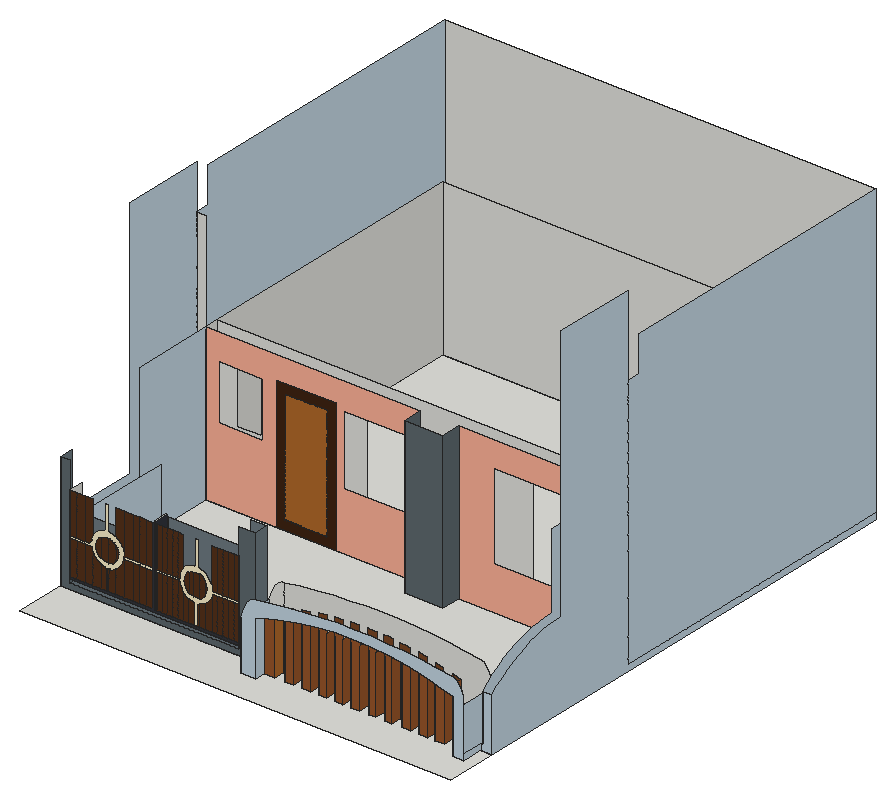
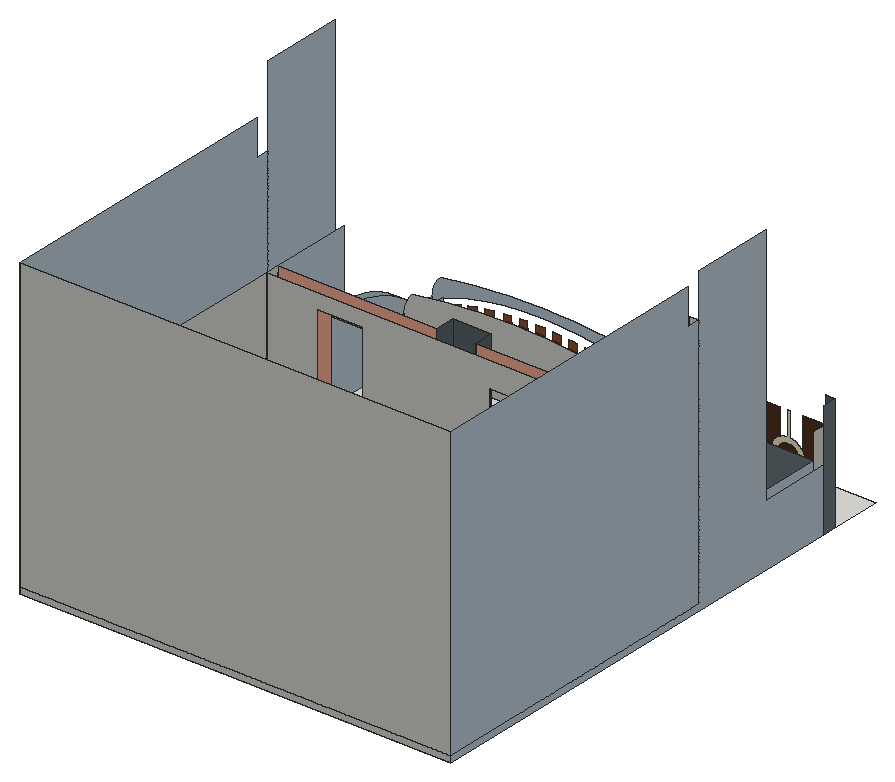
# SketchUp Ruby script. Lengths in inches.
U = 1.inch
M = Sketchup.active_model
def pt(a) = Geom::Point3d.new(a.map { |v| v * U })
def face(e, loops, mat)
  f = e.add_face(loops[0].map { |a| pt(a) })
  loops[1..].each { |l| e.add_face(l.map { |a| pt(a) }).erase! }
  f.material = f.back_material = mat if mat
  f
end
# faces: each face lists its corners as indices into pts; further lists are holes
def faces(e, pts, list, mat = nil) = list.each { |f| face(e, (f[0].is_a?(Array) ? f : [f]).map { |l| l.map { |i| pts[i] } }, mat) }
# xy, xz, yz: faces in a plane at the given z, y or x. An outline is a flat list of corners, or four numbers for a rectangle; further outlines are holes
def ring(l) = l.size == 4 ? [[l[0], l[1]], [l[2], l[1]], [l[2], l[3]], [l[0], l[3]]] : l.each_slice(2).to_a
def flat(e, list, mat, &to3) = list.each { |f| face(e, (f[0].is_a?(Array) ? f : [f]).map { |l| ring(l).map { |u, v| to3.(u, v) } }, mat) }
def xy(e, z, list, mat = nil) = flat(e, list, mat) { |x, y| [x, y, z] }
def xz(e, y, list, mat = nil) = flat(e, list, mat) { |x, z| [x, y, z] }
def yz(e, x, list, mat = nil) = flat(e, list, mat) { |y, z| [x, y, z] }
def lines(e, pts, list) = list.each { |a, b| e.add_line(pt(pts[a]), pt(pts[b])) }
# prism: a flat outline (further loops are holes) pulled along v
def prism(e, loops, v, mat = nil)
  f = face(e, loops, mat); d = Geom::Vector3d.new(v.map { |x| x * U })
  f.pushpull(f.normal.samedirection?(d) ? d.length : -d.length)
end
def box(e, o, s, mat = nil) = prism(e, [[o, [o[0] + s[0], o[1], o[2]], [o[0] + s[0], o[1] + s[1], o[2]], [o[0], o[1] + s[1], o[2]]]], [0, 0, s[2]], mat)
def at(x, y, z, deg = 0) = Geom::Transformation.translation(pt([x, y, z])) * Geom::Transformation.rotation(ORIGIN, Z_AXIS, deg.degrees)
def axes(o, x, y, z) = Geom::Transformation.new([*x, 0, *y, 0, *z, 0, *pt(o).to_a, 1])
def part(name) = M.definitions.add(name)
# library, detail: a bought-in or finely detailed component or shape, given as its bounding box
def library(name, o, s) = part(name).tap { |d| box(d.entities, o, s) }
def detail(e, o, s) = box(e.add_group.entities, o, s)
def put(e, d, t, mat = nil) = e.add_instance(d, t).tap { |i| i.material = mat if mat }
def group(e, t, mat = nil) = e.add_group.tap { |g| g.transformation = t; g.material = mat if mat }.entities
root = M.entities
M.materials.add("[Color B02]").color = [255, 178, 153]
M.materials.add("[Color D01]").color = [255, 242, 204]
M.materials.add("[Formica Laminate Dark]").color = [50, 53, 60]
M.materials.add("[Formica Speckled Grey]").color = [110, 123, 130]
M.materials.add("[Formica Speckled Grey]1").color = [94, 105, 111]
M.materials.add("[Terrazzo Light Blue]").color = [196, 214, 227]
M.materials.add("[Wood Bamboo]").color = [177, 105, 43]
M.materials.add("[Wood Cherry Original]").color = [152, 86, 42]
M.materials.add("[Wood Veneer 01]1").color = [86, 50, 26]
M.materials.add("[Wood Veneer 01]2").color = [63, 37, 19]
M.materials.add("[Wood Veneer 01]3").color = [120, 70, 37]
xy(root,0,[[0,0,0,105.19,405.48,105.19,405.48,61.94,435.4375,61.94,435.4375,84.44,457.01,84.44,457.01,105.19,477.51,105.19,477.51,84.44,495.83,84.44,495.83,105.19,513.14,105.19,513.14,84.44,530.58,84.44,530.58,105.19,547.58,105.19,547.58,84.44,564.14,84.44,564.14,105.19,580.83,105.19,580.83,84.44,597.64,84.44,597.64,105.19,613.45,105.19,613.45,84.44,631.83,84.44,631.83,105.19,650.26,105.19,650.26,84.44,665.7,84.44,665.7,105.19,683.14,105.19,683.14,84.44,698.33,84.44,698.33,105.19,718.2,105.19,718.2,84.44,736.39,84.44,736.39,105.19,754.39,105.19,754.39,84.44,771.39,84.44,771.39,105.19,787.33,105.19,787.33,84.44,806.7,84.44,806.7,105.19,823.96,105.19,823.96,84.44,841.21,84.44,841.21,61.94,863.71,61.94,863.71,105.19,887.77,105.19,887.77,0],[405.48,61.94,405.48,105.19,457.01,105.19,457.01,84.44,435.4375,84.44,435.4375,61.94],[841.21,61.94,841.21,84.44,823.96,84.44,823.96,105.19,863.71,105.19,863.71,61.94],[477.51,84.44,495.83,105.19],[513.14,84.44,530.58,105.19],
  [547.58,84.44,564.14,105.19],[580.83,84.44,597.64,105.19],[613.45,84.44,631.83,105.19],[650.26,84.44,665.7,105.19],[683.14,84.44,698.33,105.19],
  [718.2,84.44,736.39,105.19],[754.39,84.44,771.39,105.19],[787.33,84.44,806.7,105.19],[0,105.19,887.77,1092.49]])
xy(root,12.42,[[400.73,105.19,405.48,134.14],[863.71,105.19,868.09,134.14],[19.68,134.14,868.09,134.14,868.09,454.3,539.55,454.3,539.55,414.17,460.73,414.17,460.73,454.3,19.68,454.3],[460.73,414.17,539.55,414.17,539.55,454.3,868.09,454.3,868.09,482.57,258.72,482.57,258.72,454.3,460.73,454.3],[0,454.3,0,1092.49,887.77,1092.49,887.77,454.3,868.09,454.3,868.09,1063.55,19.68,1063.55,19.68,454.3],
  [19.68,454.3,177.29,482.57],[177.29,454.3,258.72,482.57],[19.68,482.57,868.09,1063.55]])
xy(root,12.42,[[19.68,105.19,367.43,134.14]],"[Formica Speckled Grey]1")
xy(root,18.66,[[19.68,105.19,367.43,134.14]])
xy(root,23.27,[[19.68,105.19,190.08,134.14],[193.18,105.19,194.95,134.14],[198.05,105.19,367.43,134.14]])
xz(root,61.94,[[405.48,0,435.4375,0,435.4375,112.74,443.36,115.36,481.41,125.65,519.59,133.66,557.87,139.38,596.21,142.82,634.59,143.96,672.97,142.82,711.32,139.38,749.6,133.66,787.78,125.65,825.83,115.36,841.21,110.27,841.21,0,863.71,0,863.71,102.81,863.19,108.38,862.36,113.8,861.24,118.99,859.83,123.88,858.16,128.43,856.24,132.55,854.11,136.22,851.78,139.36,849.3,141.96,846.6875,143.96,843.98,145.36,841.21,146.12,807.45,151.02,773.66,155.03,739.84,158.15,706.01,160.38,672.17,161.72,638.32,162.17,604.47,161.72,570.63,160.38,536.8,158.15,502.99,155.03,469.2,151.02,435.4375,146.12,432.24,145.32,429.09,143.93,426.02,141.98,423.05,139.48,420.2,136.44,417.5,132.89,414.96,128.87,412.62,124.4,410.48,119.51,408.5625,114.26,406.89,108.68,405.48,102.81]],"[Terrazzo Light Blue]")
xz(root,84.44,[[435.4375,0,457.01,0,457.01,119.05,443.36,115.36,435.4375,112.74],[477.51,0,495.83,0,495.83,128.67,481.41,125.65,477.51,124.6],[513.14,0,530.58,0,530.58,135.3,519.59,133.66,513.14,132.3],[547.58,0,564.14,0,564.14,139.94,557.87,139.38,547.58,137.84],[580.83,0,597.64,0,597.64,142.86,596.21,142.82,580.83,141.4375],
  [613.45,0,631.83,0,631.83,143.88,613.45,143.33],[650.26,0,665.7,0,665.7,143.04,650.26,143.5],[683.14,0,698.33,0,698.33,140.55,683.14,141.91],[718.2,0,736.39,0,736.39,135.63,718.2,138.35],[754.39,0,771.39,0,771.39,129.09,754.39,132.65],
  [787.33,0,806.7,0,806.7,120.53,787.78,125.65,787.33,125.74],[823.96,0,841.21,0,841.21,110.27,825.83,115.36,823.96,115.87]],"[Wood Cherry Original]")
xz(root,105.19,[[[91.99,23.27,96.375,23.27,96.375,64.97,97.1875,64.98,98,65.01,98.12,65.02,98.8125,65.06,99.62,65.125,100.43,65.21,101.24,65.32,102.04,65.45,102.84,65.59,103.64,65.76,104.43,65.94,105.21,66.14,106,66.37,106.77,66.61,107.54,66.86,108.31,67.14,109.07,67.4375,109.82,67.75,110.56,68.08,111.29,68.43,112.02,68.8,112.73,69.18,113.44,69.58,114.14,70,114.31,70.11,114.83,70.4375,115.5,70.89,116.17,71.35,116.82,71.84,117.46,72.33,118.09,72.85,118.71,73.375,119.32,73.92,119.91,74.48,120.49,75.05,121.05,75.63,121.6,76.23,122.66,77.47,123.16,78.11,123.65,78.76,124.125,79.42,124.58,80.09,125.02,80.77,125.45,81.46,125.86,82.16,126.25,82.875,126.625,83.6,126.98,84.33,127.32,85.07,127.64,85.8125,127.95,86.57,128.23,87.33,128.5,88.1,128.75,88.87,128.98,89.65,129.19,90.44,129.38,91.23,129.56,92.02,129.71,92.82,129.85,93.62,129.67,94.46,190.08,94.46,190.08,98.85,130.25,98.85,130.24,99.73,130.2,100.62,130.15,101.5,130.07,102.39,129.96,103.27,129.83,104.14,129.68,105.02,129.51,105.89,129.31,106.75,129.1,107.61,128.86,108.47,128.59,109.3125,128.31,110.15,128,110.99,127.67,111.81,127.32,112.625,126.95,113.43,126.56,114.22,126.15,115.01,125.71,115.78,125.26,116.55,124.79,117.3,124.29,118.03,123.78,118.76,123.25,119.47,122.7,120.16,122.13,120.85,121.55,121.51,120.95,122.16,120.33,122.8,119.69,123.42,119.04,124.02,118.375,124.6,117.69,125.17,117,125.72,116.29,126.25,115.5625,126.76,114.83,127.26,114.31,127.58,114.08,127.73,113.3125,128.18,112.54,128.62,111.75,129.03,110.96,129.42,110.15,129.79,109.34,130.14,108.52,130.47,107.68,130.78,106.84,131.0625,106,131.33,105.14,131.57,104.28,131.78,103.42,131.98,102.55,132.15,101.68,132.3,100.8,132.43,99.92,132.53,99.03,132.62,98.15,132.67,98.12,132.68,97.26,132.71,96.375,132.72,96.375,183.04,91.99,183.04,91.99,132.14,91.15,132.31,90.35,132.18,89.55,132.03,88.76,131.85,87.97,131.66,87.18,131.45,86.4,131.22,85.63,130.97,84.86,130.7,84.1,130.42,83.34,130.11,82.6,129.79,81.93,129.49,81.86,129.45,81.13,129.1,80.41,128.72,79.7,128.33,78.99,127.92,78.3,127.49,77.62,127.05,76.95,126.59,76.29,126.12,75.64,125.63,75,125.125,74.375,124.6,73.76,124.07,73.17,123.52,72.58,122.96,72.01,122.38,71.45,121.79,70.91,121.18,70.38,120.5625,69.87,119.93,69.37,119.29,68.88,118.64,68.42,117.97,67.97,117.3,67.53,116.61,67.11,115.91,66.71,115.2,66.33,114.49,65.96,113.76,65.75,113.31,65.61,113.03,65.28,112.29,64.97,111.54,64.67,110.78,64.39,110.01,64.14,109.24,63.9,108.47,63.67,107.68,63.47,106.9,63.29,106.11,63.125,105.31,62.98,104.51,62.85,103.71,62.74,102.9,62.66,102.09,62.59,101.28,62.54,100.47,62.51,99.66,62.5,98.85,19.68,98.85,19.68,94.46,63.08,94.46,62.9,93.69,63.02,92.96,63.15,92.24,63.3,91.51,63.47,90.79,63.85,89.37,64.07,88.66,64.3,87.96,64.54,87.26,64.8,86.57,65.08,85.88,65.37,85.2,65.67,84.53,65.75,84.38,65.99,83.86,66.33,83.2,66.68,82.55,67.04,81.91,67.42,81.27,67.81,80.64,68.21,80.03,68.63,79.42,69.06,78.81,69.5,78.22,69.96,77.64,70.43,77.07,70.91,76.51,71.4,75.96,71.91,75.42,72.42,74.89,72.95,74.375,73.49,73.87,74.04,73.375,74.6,72.9,75.17,72.43,75.75,71.97,76.35,71.53,76.95,71.1,77.56,70.68,78.17,70.28,78.8,69.89,79.4375,69.51,80.08,69.15,80.73,68.8,81.39,68.46,81.93,68.2,82.06,68.14,82.73,67.84,83.41,67.55,84.1,67.27,84.79,67.01,85.49,66.77,86.19,66.54,86.9,66.32,87.61,66.125,88.32,65.94,89.04,65.77,89.77,65.62,90.49,65.49,91.22,65.36,91.99,65.55],[96.375,75.07,93.89,75.2,91.43,75.59,89.03,76.23,86.7,77.12,84.49,78.25,82.4,79.61,81.93,79.98,80.47,81.17,78.71,82.93,77.14,84.87,75.78,86.96,74.65,89.17,73.76,91.5,73.12,93.9,72.73,96.36,72.6,98.85,72.73,101.33,73.12,103.79,73.76,106.19,74.65,108.52,75.78,110.73,77.14,112.82,78.71,114.76,80.47,116.52,81.93,117.71,82.4,118.08,84.49,119.4375,86.7,120.57,89.03,121.46,91.43,122.1,93.89,122.49,96.375,122.625,98.12,122.53,98.86,122.49,101.32,122.1,103.72,121.46,106.05,120.57,108.27,119.4375,110.35,118.08,112.29,116.52,114.05,114.76,114.31,114.43,115.61,112.82,116.97,110.73,118.1,108.52,118.99,106.19,119.63,103.79,120.02,101.33,120.15,98.85,120.02,96.36,119.63,93.9,118.99,91.5,118.1,89.17,116.97,86.96,115.61,84.87,114.31,83.26,114.05,82.93,112.29,81.17,110.35,79.61,108.27,78.25,106.05,77.12,103.72,76.23,101.32,75.59,98.86,75.2,98.12,75.16]],[[276.11,23.27,280.49,23.27,280.49,65.27,283.15,65.59,285.71,66.18,286.74,66.42,290.22,67.61,293.5625,69.17,296.72,71.0625,296.83,71.15,299.67,73.28,302.36,75.79,304.78,78.57,306.9,81.58,308.6875,84.8,310.13,88.19,310.25,88.59,311.21,91.72,311.74,94.46,367.43,94.46,367.43,98.85,312.0625,98.85,311.88,102.39,311.32,105.89,310.41,109.3125,310.25,109.72,309.13,112.625,307.53,115.78,305.59,118.76,303.36,121.51,300.86,124.02,298.1,126.25,296.83,127.07,295.125,128.18,291.97,129.79,288.66,131.0625,285.71,131.85,285.23,131.98,282.74,132.375,282.74,183.04,278.36,183.04,278.36,132.71,278.1875,132.72,274.65,132.53,274.58,132.52,271.15,131.98,267.72,131.0625,264.41,129.79,263.46,129.31,261.25,128.18,258.28,126.25,255.52,124.02,253.01,121.51,252.33,120.67,250.78,118.76,248.85,115.78,247.24,112.625,245.97,109.3125,245.05,105.89,244.5,102.39,244.3125,98.85,198.05,98.85,198.05,94.46,244.63,94.46,244.95,91.89,245.72,88.5625,246.83,85.34,248.28,82.24,250.04,79.32,252.09,76.59,252.33,76.33,254.42,74.1,257,71.86,259.8,69.9,262.78,68.25,263.46,67.96,265.93,66.92,269.19,65.92,272.54,65.27,274.58,65.09,275.94,64.98,276.11,64.98],[278.1875,75.07,275.7,75.2,274.58,75.375,273.24,75.59,270.84,76.23,268.52,77.12,266.3,78.25,264.21,79.61,263.46,80.22,262.28,81.17,260.52,82.93,258.95,84.87,257.6,86.96,256.47,89.17,255.57,91.5,254.93,93.9,254.54,96.36,254.41,98.85,254.54,101.33,254.93,103.79,255.57,106.19,256.47,108.52,257.6,110.73,258.95,112.82,260.52,114.76,262.28,116.52,263.46,117.47,264.21,118.08,266.3,119.4375,268.52,120.57,270.84,121.46,273.24,122.1,274.58,122.32,275.7,122.49,278.1875,122.625,280.67,122.49,283.13,122.1,285.54,121.46,285.71,121.39,287.86,120.57,290.08,119.4375,292.17,118.08,294.1,116.52,295.86,114.76,296.83,113.55,297.43,112.82,298.78,110.73,299.91,108.52,300.8,106.19,301.45,103.79,301.84,101.33,301.97,98.85,301.84,96.36,301.45,93.9,300.8,91.5,299.91,89.17,298.78,86.96,297.43,84.87,296.83,84.14,295.86,82.93,294.1,81.17,292.17,79.61,290.08,78.25,287.86,77.12,285.71,76.3,285.54,76.23,283.13,75.59,280.67,75.2]]],"[Color D01]")
xz(root,105.19,[[19.68,18.66,367.43,18.66,367.43,23.27,198.05,23.27,198.05,183.04,194.95,183.04,194.95,23.27,193.18,23.27,193.18,183.04,190.08,183.04,190.08,23.27,19.68,23.27]],"[Formica Laminate Dark]")
xz(root,105.19,[[0,0,405.48,0,405.48,12.42,400.73,12.42,400.73,238.16,367.43,238.16,367.43,12.42,19.68,12.42,19.68,238.16,0,238.16]],"[Formica Speckled Grey]1")
xz(root,105.19,[[863.71,0,887.77,0,887.77,109.72,868.09,108.42,868.09,12.42,863.71,12.42]],"[Terrazzo Light Blue]")
xz(root,105.19,[[19.68,23.27,33.37,94.46],[33.37,23.27,49.56,94.46],[49.56,23.27,65.75,23.27,65.75,84.38,65.67,84.53,65.37,85.2,65.08,85.88,64.8,86.57,64.54,87.26,64.3,87.96,64.07,88.66,63.85,89.37,63.47,90.79,63.3,91.51,63.15,92.24,63.02,92.96,62.9,93.69,63.08,94.46,49.56,94.46],[65.75,23.27,81.93,23.27,81.93,68.2,81.39,68.46,80.73,68.8,80.08,69.15,79.4375,69.51,78.8,69.89,78.17,70.28,77.56,70.68,76.95,71.1,76.35,71.53,75.75,71.97,75.17,72.43,74.6,72.9,74.04,73.375,73.49,73.87,72.95,74.375,72.42,74.89,71.91,75.42,71.4,75.96,70.91,76.51,70.43,77.07,69.96,77.64,69.5,78.22,69.06,78.81,68.63,79.42,68.21,80.03,67.81,80.64,67.42,81.27,67.04,81.91,66.68,82.55,66.33,83.2,65.99,83.86,65.75,84.38],[81.93,23.27,91.99,23.27,91.99,65.55,91.22,65.36,90.49,65.49,89.77,65.62,89.04,65.77,88.32,65.94,87.61,66.125,86.9,66.32,86.19,66.54,85.49,66.77,84.79,67.01,84.1,67.27,83.41,67.55,82.73,67.84,82.06,68.14,81.93,68.2],
  [96.375,23.27,98.12,23.27,98.12,65.02,98,65.01,97.1875,64.98,96.375,64.97],[98.12,23.27,114.31,23.27,114.31,70.11,114.14,70,113.44,69.58,112.73,69.18,112.02,68.8,111.29,68.43,110.56,68.08,109.82,67.75,109.07,67.4375,108.31,67.14,107.54,66.86,106.77,66.61,106,66.37,105.21,66.14,104.43,65.94,103.64,65.76,102.84,65.59,102.04,65.45,101.24,65.32,100.43,65.21,99.62,65.125,98.8125,65.06,98.12,65.02],[114.31,23.27,130.5,23.27,130.5,94.46,129.67,94.46,129.85,93.62,129.71,92.82,129.56,92.02,129.38,91.23,129.19,90.44,128.98,89.65,128.75,88.87,128.5,88.1,128.23,87.33,127.95,86.57,127.64,85.8125,127.32,85.07,126.98,84.33,126.625,83.6,126.25,82.875,125.86,82.16,125.45,81.46,125.02,80.77,124.58,80.09,124.125,79.42,123.65,78.76,123.16,78.11,122.66,77.47,121.6,76.23,121.05,75.63,120.49,75.05,119.91,74.48,119.32,73.92,118.71,73.375,118.09,72.85,117.46,72.33,116.82,71.84,116.17,71.35,115.5,70.89,114.83,70.4375,114.31,70.11],[130.5,23.27,147.75,94.46],[147.75,23.27,161.81,94.46],
  [161.81,23.27,175.94,94.46],[175.94,23.27,190.08,94.46],[198.05,23.27,207.83,94.46],[207.83,23.27,218.96,94.46],[218.96,23.27,230.08,94.46],
  [230.08,23.27,241.21,94.46],[241.21,23.27,252.33,23.27,252.33,76.33,252.09,76.59,250.04,79.32,248.28,82.24,246.83,85.34,245.72,88.5625,244.95,91.89,244.63,94.46,241.21,94.46],[252.33,23.27,263.46,23.27,263.46,67.96,262.78,68.25,259.8,69.9,257,71.86,254.42,74.1,252.33,76.33],[263.46,23.27,274.58,23.27,274.58,65.09,272.54,65.27,269.19,65.92,265.93,66.92,263.46,67.96],[274.58,23.27,276.11,23.27,276.11,64.98,275.94,64.98,274.58,65.09],
  [280.49,23.27,285.71,23.27,285.71,66.18,283.15,65.59,280.49,65.27],[285.71,23.27,296.83,23.27,296.83,71.15,296.72,71.0625,293.5625,69.17,290.22,67.61,286.74,66.42,285.71,66.18],[296.83,23.27,310.25,23.27,310.25,88.59,310.13,88.19,308.6875,84.8,306.9,81.58,304.78,78.57,302.36,75.79,299.67,73.28,296.83,71.15],[310.25,23.27,321.7,23.27,321.7,94.46,311.74,94.46,311.21,91.72,310.25,88.59],[321.7,23.27,333.57,94.46],
  [333.57,23.27,343.875,94.46],[343.875,23.27,355.65,94.46],[355.65,23.27,367.43,94.46],[96.375,75.07,98.12,75.16,98.12,122.53,96.375,122.625,93.89,122.49,91.43,122.1,89.03,121.46,86.7,120.57,84.49,119.4375,82.4,118.08,81.93,117.71,81.93,79.98,82.4,79.61,84.49,78.25,86.7,77.12,89.03,76.23,91.43,75.59,93.89,75.2],[278.1875,75.07,280.67,75.2,283.13,75.59,285.54,76.23,285.71,76.3,285.71,121.39,285.54,121.46,283.13,122.1,280.67,122.49,278.1875,122.625,275.7,122.49,274.58,122.32,274.58,75.375,275.7,75.2],
  [98.12,75.16,98.86,75.2,101.32,75.59,103.72,76.23,106.05,77.12,108.27,78.25,110.35,79.61,112.29,81.17,114.05,82.93,114.31,83.26,114.31,114.43,114.05,114.76,112.29,116.52,110.35,118.08,108.27,119.4375,106.05,120.57,103.72,121.46,101.32,122.1,98.86,122.49,98.12,122.53],[274.58,75.375,274.58,122.32,273.24,122.1,270.84,121.46,268.52,120.57,266.3,119.4375,264.21,118.08,263.46,117.47,263.46,80.22,264.21,79.61,266.3,78.25,268.52,77.12,270.84,76.23,273.24,75.59],[285.71,76.3,287.86,77.12,290.08,78.25,292.17,79.61,294.1,81.17,295.86,82.93,296.83,84.14,296.83,113.55,295.86,114.76,294.1,116.52,292.17,118.08,290.08,119.4375,287.86,120.57,285.71,121.39],[81.93,79.98,81.93,117.71,80.47,116.52,78.71,114.76,77.14,112.82,75.78,110.73,74.65,108.52,73.76,106.19,73.12,103.79,72.73,101.33,72.6,98.85,72.73,96.36,73.12,93.9,73.76,91.5,74.65,89.17,75.78,86.96,77.14,84.87,78.71,82.93,80.47,81.17],[263.46,80.22,263.46,117.47,262.28,116.52,260.52,114.76,258.95,112.82,257.6,110.73,256.47,108.52,255.57,106.19,254.93,103.79,254.54,101.33,254.41,98.85,254.54,96.36,254.93,93.9,255.57,91.5,256.47,89.17,257.6,86.96,258.95,84.87,260.52,82.93,262.28,81.17],
  [114.31,83.26,115.61,84.87,116.97,86.96,118.1,89.17,118.99,91.5,119.63,93.9,120.02,96.36,120.15,98.85,120.02,101.33,119.63,103.79,118.99,106.19,118.1,108.52,116.97,110.73,115.61,112.82,114.31,114.43],[296.83,84.14,297.43,84.87,298.78,86.96,299.91,89.17,300.8,91.5,301.45,93.9,301.84,96.36,301.97,98.85,301.84,101.33,301.45,103.79,300.8,106.19,299.91,108.52,298.78,110.73,297.43,112.82,296.83,113.55],[19.68,98.85,33.37,183.04],[33.37,98.85,49.56,183.04],[49.56,98.85,62.5,98.85,62.51,99.66,62.54,100.47,62.59,101.28,62.66,102.09,62.74,102.9,62.85,103.71,62.98,104.51,63.125,105.31,63.29,106.11,63.47,106.9,63.67,107.68,63.9,108.47,64.14,109.24,64.39,110.01,64.67,110.78,64.97,111.54,65.28,112.29,65.61,113.03,65.75,113.31,65.75,183.04,49.56,183.04],
  [130.25,98.85,130.5,98.85,130.5,183.04,114.31,183.04,114.31,127.58,114.83,127.26,115.5625,126.76,116.29,126.25,117,125.72,117.69,125.17,118.375,124.6,119.04,124.02,119.69,123.42,120.33,122.8,120.95,122.16,121.55,121.51,122.13,120.85,122.7,120.16,123.25,119.47,123.78,118.76,124.29,118.03,124.79,117.3,125.26,116.55,125.71,115.78,126.15,115.01,126.56,114.22,126.95,113.43,127.32,112.625,127.67,111.81,128,110.99,128.31,110.15,128.59,109.3125,128.86,108.47,129.1,107.61,129.31,106.75,129.51,105.89,129.68,105.02,129.83,104.14,129.96,103.27,130.07,102.39,130.15,101.5,130.2,100.62,130.24,99.73],[130.5,98.85,147.75,183.04],[147.75,98.85,161.81,183.04],[161.81,98.85,175.94,183.04],[175.94,98.85,190.08,183.04],
  [198.05,98.85,207.83,183.04],[207.83,98.85,218.96,183.04],[218.96,98.85,230.08,183.04],[230.08,98.85,241.21,183.04],[241.21,98.85,244.3125,98.85,244.5,102.39,245.05,105.89,245.97,109.3125,247.24,112.625,248.85,115.78,250.78,118.76,252.33,120.67,252.33,183.04,241.21,183.04],
  [312.0625,98.85,321.7,98.85,321.7,183.04,310.25,183.04,310.25,109.72,310.41,109.3125,311.32,105.89,311.88,102.39],[321.7,98.85,333.57,183.04],[333.57,98.85,343.875,183.04],[343.875,98.85,355.65,183.04],[355.65,98.85,367.43,183.04]],"[Wood Veneer 01]1")
xz(root,105.19,[[457.01,0,477.51,0,477.51,124.6,457.01,119.05],[495.83,0,513.14,0,513.14,132.3,495.83,128.67],[530.58,0,547.58,0,547.58,137.84,530.58,135.3],[564.14,0,580.83,0,580.83,141.4375,564.14,139.94],[597.64,0,613.45,0,613.45,143.33,597.64,142.86],
  [631.83,0,650.26,0,650.26,143.5,634.59,143.96,631.83,143.88],[665.7,0,683.14,0,683.14,141.91,672.97,142.82,665.7,143.04],[698.33,0,718.2,0,718.2,138.35,711.32,139.38,698.33,140.55],[736.39,0,754.39,0,754.39,132.65,749.6,133.66,736.39,135.63],[771.39,0,787.33,0,787.33,125.74,771.39,129.09],
  [806.7,0,823.96,0,823.96,115.87,806.7,120.53]],"[Wood Veneer 01]3")
xz(root,134.14,[[405.48,12.42,405.48,102.81,406.89,108.68,408.5625,114.26,410.48,119.51,412.62,124.4,414.96,128.87,417.5,132.89,420.2,136.44,423.05,139.48,426.02,141.98,429.09,143.93,432.24,145.32,435.4375,146.12,435.4375,12.42],[435.4375,12.42,435.4375,146.12,469.2,151.02,502.99,155.03,536.8,158.15,570.63,160.38,604.47,161.72,638.32,162.17,672.17,161.72,706.01,160.38,739.84,158.15,773.66,155.03,807.45,151.02,841.21,146.12,843.98,145.36,846.6875,143.96,849.3,141.96,851.78,139.36,854.11,136.22,856.24,132.55,858.16,128.43,859.83,123.88,861.24,118.99,862.36,113.8,863.19,108.38,863.71,102.81,863.71,12.42],[19.68,18.66,19.68,23.27,190.08,23.27,190.08,183.04,193.18,183.04,193.18,23.27,194.95,23.27,194.95,183.04,198.05,183.04,198.05,23.27,367.43,23.27,367.43,18.66]])
xz(root,134.14,[[367.43,12.42,400.73,238.16],[19.68,23.27,190.08,128.61],[198.05,23.27,367.43,183.04]],"[Formica Speckled Grey]")
xz(root,414.17,[[460.73,12.42,539.55,330.6]],"[Formica Speckled Grey]1")
xz(root,454.3,[[0,12.42,19.68,535.72]])
xz(root,454.3,[[[19.68,12.42,163.18,12.42,163.18,284.17,288.36,284.17,288.36,12.42,460.73,12.42,460.73,330.6,19.68,330.6],[303.04,131.32,430.98,275.13],[45.16,162.09,136.97,276.9]],[[539.55,12.42,868.09,330.6],[611.1,100.57,757.91,278.13]]],"[Color B02]")
xz(root,454.3,[[182.5,31.74,269.05,264.85]],"[Wood Bamboo]")
xz(root,454.3,[[[163.18,12.42,288.36,284.17],[182.5,31.74,269.05,264.85]]],"[Wood Veneer 01]2")
xz(root,482.57,[[[19.68,12.42,19.68,330.6,868.09,330.6,868.09,12.42,258.72,12.42,258.72,279.81,177.29,279.81,177.29,12.42],[669.05,74.49,764.12,300.55],[328.38,90.05,411.43,279.11],[61.14,149.35,112.95,294.68]]])
xz(root,1063.55,[[19.68,12.42,868.09,330.6]])
xz(root,1092.49,[[0,0,887.77,12.42],[0,12.42,887.77,609.41]])
yz(root,0,[[105.19,0,134.14,238.16]],"[Formica Speckled Grey]")
yz(root,0,[[134.14,0,134.14,128.61,283.27,128.61,283.27,627.66,454.3,627.66,454.3,12.42,1092.49,12.42,1092.49,0],[454.3,12.42,454.3,535.72,482.57,535.72,482.57,609.41,1092.49,609.41,1092.49,12.42]],"[Terrazzo Light Blue]")
yz(root,19.68,[[454.3,12.42,482.57,330.6],[482.57,12.42,1063.55,330.6],[105.19,18.66,134.14,23.27],[105.19,23.27,134.14,183.04]])
yz(root,19.68,[[105.19,12.42,134.14,18.66]],"[Formica Speckled Grey]1")
yz(root,19.68,[[134.14,12.42,340.77,128.61],[340.77,12.42,454.3,12.42,454.3,330.6,283.27,330.6,283.27,128.61,340.77,128.61]],"[Terrazzo Light Blue]")
yz(root,193.18,[[105.19,23.27,134.14,186.5625]])
yz(root,194.95,[[105.19,23.27,134.14,186.5625]],"[Formica Laminate Dark]")
yz(root,367.43,[[105.19,18.66,134.14,21.55],[105.19,23.27,134.14,183.04]])
yz(root,367.43,[[105.19,12.42,134.14,18.66]],"[Formica Speckled Grey]1")
yz(root,400.73,[[105.19,12.42,134.14,238.16]],"[Formica Speckled Grey]")
yz(root,405.48,[[61.94,0,105.19,12.42],[61.94,12.42,134.14,102.81]],"[Terrazzo Light Blue]")
yz(root,435.4375,[[61.94,0,84.44,112.74]],"[Terrazzo Light Blue]")
yz(root,457.01,[[84.44,0,105.19,119.05]],"[Wood Bamboo]")
yz(root,460.73,[[414.17,12.42,454.3,330.6]],"[Formica Speckled Grey]1")
yz(root,477.51,[[84.44,0,105.19,119.05]],"[Wood Cherry Original]")
yz(root,495.83,[[84.44,0,105.19,119.05]],"[Wood Cherry Original]")
yz(root,513.14,[[84.44,0,105.19,119.05]],"[Wood Cherry Original]")
yz(root,530.58,[[84.44,0,105.19,119.05]],"[Wood Cherry Original]")
yz(root,539.55,[[414.17,12.42,454.3,330.6]],"[Formica Speckled Grey]1")
yz(root,547.58,[[84.44,0,105.19,119.05]],"[Wood Cherry Original]")
yz(root,564.14,[[84.44,0,105.19,119.05]],"[Wood Cherry Original]")
yz(root,580.83,[[84.44,0,105.19,119.05]],"[Wood Cherry Original]")
yz(root,597.64,[[84.44,0,105.19,119.05]],"[Wood Cherry Original]")
yz(root,613.45,[[84.44,0,105.19,119.05]],"[Wood Cherry Original]")
yz(root,631.83,[[84.44,0,105.19,119.05]],"[Wood Cherry Original]")
yz(root,650.26,[[84.44,0,105.19,119.05]],"[Wood Cherry Original]")
yz(root,665.7,[[84.44,0,105.19,119.05]],"[Wood Cherry Original]")
yz(root,683.14,[[84.44,0,105.19,119.05]],"[Wood Cherry Original]")
yz(root,698.33,[[84.44,0,105.19,119.05]],"[Wood Cherry Original]")
yz(root,718.2,[[84.44,0,105.19,119.05]],"[Wood Cherry Original]")
yz(root,736.39,[[84.44,0,105.19,119.05]],"[Wood Cherry Original]")
yz(root,754.39,[[84.44,0,105.19,119.05]],"[Wood Cherry Original]")
yz(root,771.39,[[84.44,0,105.19,119.05]],"[Wood Cherry Original]")
yz(root,787.33,[[84.44,0,105.19,119.05]],"[Wood Cherry Original]")
yz(root,806.7,[[84.44,0,105.19,119.05]],"[Wood Cherry Original]")
yz(root,823.96,[[84.44,0,105.19,115.87]],"[Wood Cherry Original]")
yz(root,841.21,[[61.94,0,84.44,110.27]],"[Terrazzo Light Blue]")
yz(root,863.71,[[61.94,0,105.19,12.42],[61.94,12.42,134.14,102.81]],"[Terrazzo Light Blue]")
yz(root,868.09,[[454.3,12.42,482.57,330.6],[482.57,12.42,1063.55,330.6]])
yz(root,868.09,[[105.19,12.42,105.19,108.42,107.97,110.74,118.54,119.63,130.3,128.41,132.61,130.03,146.79,138.86,161.26,146.78,175.97,153.77,190.91,159.82,206.02,164.92,221.29,169.05,236.6875,172.21,252.17,174.38,267.71,175.57,283.27,175.78,283.27,330.6,454.3,330.6,454.3,12.42]],"[Terrazzo Light Blue]")
yz(root,887.77,[[105.19,0,1092.49,0,1092.49,12.42,454.3,12.42,454.3,702.66,283.27,702.66,283.27,175.78,267.71,175.57,252.17,174.38,236.6875,172.21,221.29,169.05,206.02,164.92,190.91,159.82,175.97,153.77,161.26,146.78,146.79,138.86,132.61,130.03,118.73,120.31,105.19,109.72],[454.3,12.42,1092.49,12.42,1092.49,609.41,482.57,609.41,482.57,535.72,454.3,535.72]],"[Terrazzo Light Blue]")
p = [[411.43,454.3,90.05],[411.43,482.57,90.05],[328.38,454.3,90.05],[328.38,482.57,90.05],[669.05,454.3,74.49],[669.05,482.57,74.49],
  [764.12,454.3,74.49],[764.12,482.57,74.49]]
lines(root,p,[[0,1],[2,3],[4,5],[6,7]])
